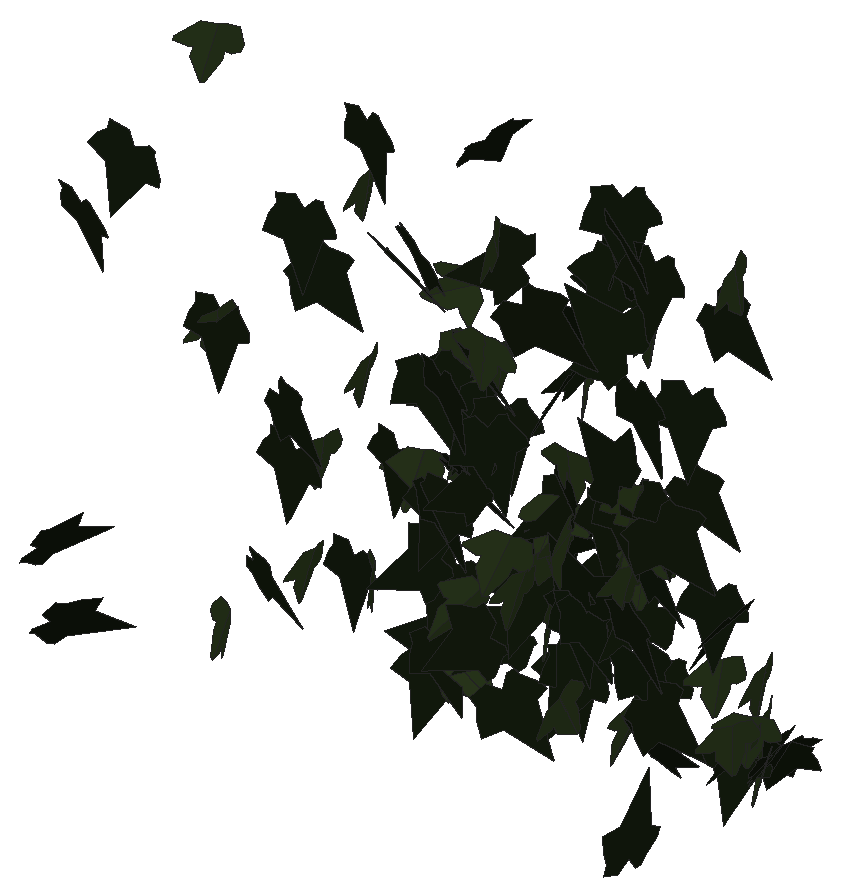
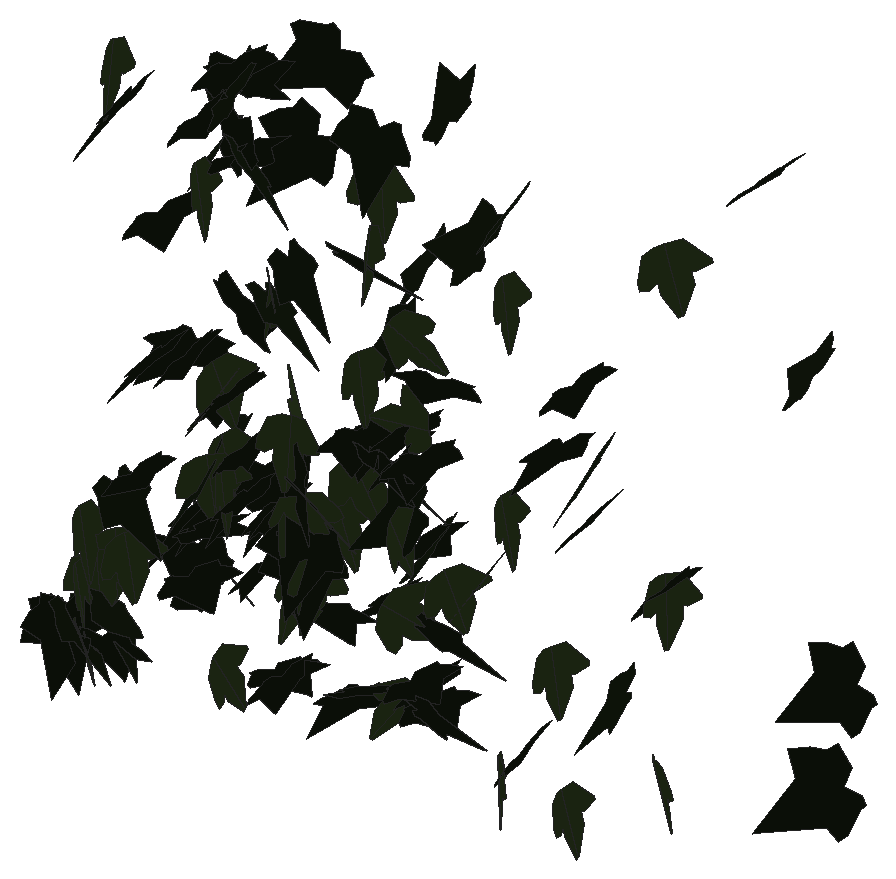
# SketchUp Ruby script. Lengths in inches.
U = 1.inch
M = Sketchup.active_model
def pt(a) = Geom::Point3d.new(a.map { |v| v * U })
def face(e, loops, mat)
  f = e.add_face(loops[0].map { |a| pt(a) })
  loops[1..].each { |l| e.add_face(l.map { |a| pt(a) }).erase! }
  f.material = f.back_material = mat if mat
  f
end
# faces: each face lists its corners as indices into pts; further lists are holes
def faces(e, pts, list, mat = nil) = list.each { |f| face(e, (f[0].is_a?(Array) ? f : [f]).map { |l| l.map { |i| pts[i] } }, mat) }
# xy, xz, yz: faces in a plane at the given z, y or x. An outline is a flat list of corners, or four numbers for a rectangle; further outlines are holes
def ring(l) = l.size == 4 ? [[l[0], l[1]], [l[2], l[1]], [l[2], l[3]], [l[0], l[3]]] : l.each_slice(2).to_a
def flat(e, list, mat, &to3) = list.each { |f| face(e, (f[0].is_a?(Array) ? f : [f]).map { |l| ring(l).map { |u, v| to3.(u, v) } }, mat) }
def xy(e, z, list, mat = nil) = flat(e, list, mat) { |x, y| [x, y, z] }
def xz(e, y, list, mat = nil) = flat(e, list, mat) { |x, z| [x, y, z] }
def yz(e, x, list, mat = nil) = flat(e, list, mat) { |y, z| [x, y, z] }
def lines(e, pts, list) = list.each { |a, b| e.add_line(pt(pts[a]), pt(pts[b])) }
# prism: a flat outline (further loops are holes) pulled along v
def prism(e, loops, v, mat = nil)
  f = face(e, loops, mat); d = Geom::Vector3d.new(v.map { |x| x * U })
  f.pushpull(f.normal.samedirection?(d) ? d.length : -d.length)
end
def box(e, o, s, mat = nil) = prism(e, [[o, [o[0] + s[0], o[1], o[2]], [o[0] + s[0], o[1] + s[1], o[2]], [o[0], o[1] + s[1], o[2]]]], [0, 0, s[2]], mat)
def at(x, y, z, deg = 0) = Geom::Transformation.translation(pt([x, y, z])) * Geom::Transformation.rotation(ORIGIN, Z_AXIS, deg.degrees)
def axes(o, x, y, z) = Geom::Transformation.new([*x, 0, *y, 0, *z, 0, *pt(o).to_a, 1])
def part(name) = M.definitions.add(name)
# library, detail: a bought-in or finely detailed component or shape, given as its bounding box
def library(name, o, s) = part(name).tap { |d| box(d.entities, o, s) }
def detail(e, o, s) = box(e.add_group.entities, o, s)
def put(e, d, t, mat = nil) = e.add_instance(d, t).tap { |i| i.material = mat if mat }
def group(e, t, mat = nil) = e.add_group.tap { |g| g.transformation = t; g.material = mat if mat }.entities
root = M.entities
M.materials.add("efeu1").color = [18, 25, 13]
M.materials.add("efeu2").color = [43, 57, 29]
c1 = part("ivyleaf_9")
p = [[1.54,2.16,1.25],[1.36,2.04,1.19],[-0.21,0.99,0.68],[-0.71,1.11,0.82],[-0.85,0.86,0.67],[-0.8,0.17,0.21],
  [-0.9,-0.01,0.1],[-0.67,-0.16,-0.02],[-0.08,-0.08,-0.05],[-0.03,-0.6,-0.4],[0.65,-0.88,-0.66],[0.83,-0.6,-0.49],
  [1.29,-0.42,-0.43],[1.8125,-0.07,-0.26],[1.21,0.44,0.15]]
faces(c1.entities,p,[[0,1,2,3,4,5,6,7,8,9,10,11,12,13,14]],"efeu1")
c2 = part("ivyleaf_10")
p = [[0,0.5,-0.03],[-0.0625,2.02,-0.43],[-0.19,2.01,-0.46],[-0.54,1.05,-0.29],[-0.52,0.625,-0.18],[-0.83,0.76,-0.28],
  [-1.16,0.64,-0.33],[-1.15,0.33,-0.24],[-0.77,-0.39,0.02],[-0.3,-0.51,0.16],[0.04,-0.48,0.23],[-0.02,2.01,-0.4375],
  [-0.06,2.01,-0.43],[0.04,-0.49,0.23],[0.67,-0.49,0.14],[1.38,0.36,-0.2],[1.375,0.51,-0.24],[0.81,0.65,-0.19],
  [0.62,0.59,-0.15],[0.6,1.09,-0.28],[0.5,1.23,-0.31]]
faces(c2.entities,p,[[0,1,2,3,4,5,6,7,8,9,10],[11,12,0,13,14,15,16,17,18,19,20]],"efeu2")
put(root,c1,axes([509.26,117.63,280.6],[0.7162,0.6229,0.94932],[0.53942,0.78067,-0.93141],[-1.06464,0.81457,0.1667]))
put(root,c1,axes([509.12,118.66,276.5],[0.94706,0.62855,0.77207],[0.59178,0.50664,-1.11926],[-0.868,1.03121,0.0793]))
put(root,c1,axes([509.17,120.39,295.65],[0.43222,-0.99904,0.53344],[0.29536,-0.45177,-1.08541],[1.09334,0.51698,0.08234]))
put(root,c2,axes([511.24,126.79,288.2],[-0.26325,-1.11937,-0.16844],[0.01435,0.16962,-1.14964],[1.13188,-0.26249,-0.0246]))
put(root,c1,axes([511.24,127.07,288.25],[0.01342,-1.16177,0.09011],[0.00969,-0.09,-1.16182],[1.16522,0.01413,0.00862]))
put(root,c2,axes([511.91,125.92,302.36],[-0.76297,-0.8833,0.30452],[-0.11819,-0.29874,-1.16269],[0.92681,-0.76525,0.10241]))
put(root,c1,axes([514.13,117.63,301.27],[-0.31009,-1.11283,0.47862],[0.13916,-0.5235,-1.12703],[1.20337,-0.22622,0.25366]))
put(root,c2,axes([514.92,122.69,276.87],[0.81565,-0.77415,-0.31621],[-0.18054,0.26829,-1.1225],[0.81652,0.83264,0.06768]))
put(root,c2,axes([515.36,127.93,277.68],[0.10975,-1.12799,0.06776],[0.00312,-0.06778,-1.13331],[1.13001,0.10974,-0.00345]))
put(root,c2,axes([516.27,127.56,283.53],[-0.20922,-1.13014,-0.01788],[-0.00453,0.01902,-1.14932],[1.13028,-0.20912,-0.00792]))
put(root,c1,axes([516.34,126.24,295.27],[-0.07104,-1.18727,-0.06644],[-0.00655,0.06695,-1.18934],[1.18911,-0.07057,-0.01052]))
put(root,c1,axes([516.54,122.875,279.96],[0.98177,-0.54869,-0.35898],[-0.27032,0.25016,-1.12167],[0.59737,1.01497,0.0824]))
put(root,c1,axes([516.66,126.62,292.67],[0.34915,-0.86934,-0.72445],[0.05079,0.76942,-0.89883],[1.13049,0.23392,0.26412]))
put(root,c1,axes([518.02,127.5,278.76],[0.17028,-1.0878,0.30446],[0.00985,-0.30645,-1.10045],[1.12956,0.16666,-0.0363]))
put(root,c2,axes([518.54,128.03,278.09],[0.66528,-0.87205,-0.28529],[0.0238,0.36868,-1.07143],[0.91722,0.62295,0.23473]))
put(root,c1,axes([518.7,121.82,289.12],[0.802,-0.75694,-0.50991],[-0.33518,0.3871,-1.10181],[0.84889,0.86797,0.04671]))
put(root,c2,axes([519.31,126.79,288.87],[0.23325,-1.14394,-0.09887],[-0.01611,0.09762,-1.16747],[1.14809,0.23378,0.0037]))
put(root,c1,axes([518.96,122.34,286.43],[-0.01682,-1.13373,0.40994],[0.11146,-0.40968,-1.12845],[1.2004,0.02215,0.11053]))
put(root,c2,axes([519.83,126.11,298.18],[0.19813,-1.16682,-0.20693],[-0.00093,0.20965,-1.18304],[1.18502,0.19525,0.03367]))
put(root,c1,axes([520.31,125.55,301.18],[0.43787,-1.1213,0.19248],[0.0419,-0.19021,-1.20339],[1.13693,0.43887,-0.02978]))
put(root,c1,axes([520.65,127.15,284.92],[0.11977,-1.02798,0.52313],[0.08685,-0.51641,-1.03466],[1.15016,0.14604,0.02366]))
put(root,c2,axes([521.81,127.17,284.89],[-0.57252,-0.9368,0.37642],[0.00691,-0.43636,-1.07545],[1.00957,-0.52826,0.22083]))
put(root,c1,axes([523.875,125.76,281.52],[-1.13577,0.158,0.39255],[-0.39229,0.02835,-1.14644],[-0.15863,-1.20136,0.02457]))
put(root,c1,axes([524.3,125.875,277.77],[-0.76854,0.43127,0.72687],[-0.6887,0.24993,-0.87647],[-0.48992,-1.02787,0.09185]))
put(root,c1,axes([523.35,127.53,280.19],[-0.45479,-1.05416,0.10034],[-0.0168,-0.102,-1.14781],[1.05879,-0.45442,0.02489]))
put(root,c1,axes([523.58,126.76,289.78],[-0.13333,-1.08675,-0.43796],[0.06968,0.43265,-1.09479],[1.1696,-0.14967,0.0153]))
put(root,c2,axes([524.9,126.27,294.68],[0.60536,0.03725,-1.03146],[-1.0202,0.2029,-0.59142],[0.15649,1.17864,0.13441]))
put(root,c1,axes([524.06,125.26,284.99],[0.67213,-1.01656,-0.05675],[-0.03339,0.04595,-1.21867],[1.0176,0.67296,-0.0025]))
put(root,c1,axes([523.74,122.79,297.39],[0.80288,-0.77938,0.55092],[0.51517,-0.25216,-1.10751],[0.80346,0.9405,0.1596]))
put(root,c2,axes([523.86,126.54,290.9375],[0.14036,0.03807,1.1742],[1.14694,0.25168,-0.14526],[-0.25444,1.15547,-0.00704]))
put(root,c2,axes([524.73,126.8,286.04],[0.2892,-1.04183,0.45253],[0.21949,-0.40691,-1.07707],[1.11446,0.3505,0.0947]))
put(root,c1,axes([524.32,126.5,290.7],[0.26155,-1.05452,-0.46703],[0.08644,0.49547,-1.07032],[1.15007,0.20258,0.18666]))
put(root,c1,axes([524.8,124.69,277.38],[-0.51302,-1.02415,0.01667],[-0.00704,-0.01512,-1.14546],[1.02427,-0.51307,0.00047]))
put(root,c1,axes([524.79,125.33,284.85],[-0.40551,-1.05086,0.29037],[-0.04899,-0.29193,-1.12492],[1.08914,-0.40439,0.05751]))
put(root,c1,axes([524.74,124.68,278.42],[0.24565,-1.06693,-0.34846],[-0.01246,0.35409,-1.09296],[1.12232,0.23746,0.06413]))
put(root,c1,axes([524.85,126.5,289.15],[0.12997,-1.16541,0.11002],[-0.01541,-0.11239,-1.17231],[1.17049,0.12793,-0.02765]))
put(root,c1,axes([524.79,124.22,291.67],[-0.36293,-0.93566,-0.71448],[0.73159,0.40652,-0.90398],[0.92234,-0.69061,0.43588]))
put(root,c1,axes([524.88,125.5,286.4],[1.16623,-0.32753,0.1954],[0.18385,-0.06798,-1.21125],[0.33415,1.18053,-0.01554]))
put(root,c1,axes([525.95,126.73,288.97],[-1.14286,-0.09267,-0.27996],[0.27902,0.02292,-1.14661],[0.09547,-1.17642,-0.00028]))
put(root,c2,axes([526.34,124.9,281.04],[-0.20033,-0.71324,0.96606],[-0.16303,-0.95419,-0.73828],[1.18971,-0.25086,0.0615]))
put(root,c2,axes([525.7,124.82,277.52],[0.4045,0.81164,0.72364],[0.33338,0.64234,-0.90681],[-1.03502,0.5241,-0.00927]))
put(root,c1,axes([526.79,127.25,278.38],[-0.94856,-0.49486,0.40687],[-0.13977,-0.54959,-0.99429],[0.62521,-0.87365,0.39501]))
put(root,c1,axes([526.74,125.47,302.7],[0.22673,1.19784,0.11087],[0.00467,0.11195,-1.219],[-1.20295,0.2262,0.01617]))
put(root,c1,axes([527.5,124.24,287.05],[-1.05091,0.44694,0.30048],[-0.28768,0.09112,-1.14167],[-0.45528,-1.08922,0.02779]))
put(root,c2,axes([526.95,126.25,292.39],[-0.09969,-1.18923,-0.09221],[0.01442,0.09133,-1.19339],[1.19272,-0.10051,0.00672]))
put(root,c2,axes([526.87,125.71,297.79],[0.39208,-1.0027,-0.54799],[0.03963,0.59093,-1.05292],[1.14198,0.32375,0.22468]))
put(root,c1,axes([526.34,124.44,293.24],[1.07571,-0.63641,-0.05333],[-0.04129,0.03493,-1.24984],[0.6373,1.07647,0.00903]))
put(root,c1,axes([527.97,126,296.88],[-1.01227,0.41714,0.51111],[-0.56307,-0.0585,-1.06745],[-0.34378,-1.13247,0.24341]))
put(root,c1,axes([527.1,126.27,289.44],[-0.26345,-1.07919,-0.40375],[0.10752,0.38934,-1.11082],[1.14722,-0.28432,0.01139]))
put(root,c1,axes([527.12,125.1,289.08],[-0.06933,-1.12895,-0.51525],[0.0311,0.51431,-1.13108],[1.24058,-0.07599,-0.00044]))
put(root,c1,axes([528.2,123.63,280.21],[-0.74453,-0.56698,0.78751],[-0.29754,-0.8114,-0.86549],[0.92364,-0.71842,0.35599]))
put(root,c1,axes([528.22,127,281.4375],[-0.86515,-0.74424,-0.24341],[0.27689,0.04853,-1.13253],[0.73245,-0.89743,0.14062]))
put(root,c1,axes([528.01,125.03,276.95],[0.2607,-0.89498,-0.76674],[0.20088,0.80754,-0.87429],[1.16126,0.06123,0.32337]))
put(root,c2,axes([528.68,126.96,282.85],[-0.33954,-1.03795,-0.42553],[0.12465,0.40694,-1.09205],[1.11485,-0.36162,-0.0075]))
put(root,c1,axes([527.97,119.51,300.22],[0.05578,-0.72625,1.04556],[0.47712,-0.95836,-0.69113],[1.18026,0.42174,0.22998]))
put(root,c1,axes([529.02,126.89,283.72],[0.49402,0.99682,-0.37978],[-0.13002,-0.35914,-1.11178],[-1.05876,0.50922,-0.04068]))
put(root,c1,axes([528.19,120.66,293.93],[0.55752,-1.04352,0.42032],[0.16487,-0.38825,-1.18259],[1.11285,0.58031,-0.03537]))
put(root,c1,axes([529.07,126.73,284.24],[0.68796,0.94268,-0.15589],[-0.11006,-0.11263,-1.16681],[-0.94913,0.69635,0.02231]))
put(root,c2,axes([529.47,126.7,285.44],[1.00994,0.49951,-0.35423],[-0.42659,0.08373,-1.09817],[-0.43933,1.06698,0.25201]))
put(root,c1,axes([530.01,126.53,286],[-1.11043,0.40907,0.08257],[-0.09083,-0.00782,-1.18275],[-0.40731,-1.11347,0.03864]))
put(root,c2,axes([529.69,123.08,285.35],[-0.81779,-0.78869,0.50414],[-0.22618,-0.48311,-1.12269],[0.90832,-0.83039,0.17434]))
put(root,c1,axes([530.1,126.55,287.15],[0.29638,0.01036,-1.15019],[-1.15016,0.01616,-0.29623],[0.01307,1.18766,0.01407]))
put(root,c2,axes([529.94,123.68,283.52],[0.00108,-1.16186,0.1635],[0.0034,-0.1635,-1.16186],[1.1733,0.00155,0.00322]))
put(root,c2,axes([529.97,126.73,284.53],[0.05845,-1.17459,0.00428],[-0.01828,-0.00519,-1.1759],[1.17445,0.05838,-0.01852]))
put(root,c1,axes([529.89,127.47,278.06],[0.00002,-1.13828,-0.18638],[-0.00846,0.18637,-1.13825],[1.15341,0.00139,-0.00835]))
put(root,c2,axes([530.51,126.37,288.34],[-1.17928,-0.06347,0.16864],[-0.16845,-0.00821,-1.18099],[0.06399,-1.19125,-0.00085]))
put(root,c1,axes([530.4,127.21,278.04],[-0.69121,-0.91987,0.0399],[0.04961,-0.08703,-1.14695],[0.9194,-0.68687,0.09189]))
put(root,c2,axes([530.92,120.2,296.68],[-1.17467,-0.14325,0.28175],[-0.27014,-0.10795,-1.18116],[0.1641,-1.20316,0.07243]))
put(root,c2,axes([530.68,124.92,282.23],[0.62617,-0.91261,0.47756],[0.35083,-0.3365,-1.10304],[0.96842,0.71199,0.09081]))
put(root,c1,axes([531.9375,125.8,293.63],[-0.81161,0.89778,0.03497],[-0.14537,-0.08472,-1.19902],[-0.88663,-0.80793,0.16458]))
put(root,c1,axes([531.16,127.02,282.49],[0.27296,-1.11304,-0.23533],[-0.00022,0.24196,-1.14464],[1.13765,0.26711,0.05624]))
put(root,c1,axes([532.49,123.75,294.1],[-0.6893,0.92152,-0.45373],[0.25844,-0.37326,-1.15069],[-0.99412,-0.73599,0.01546]))
put(root,c2,axes([531.98,125.73,293.66],[-0.59366,0.84866,-0.62841],[0.03235,-0.70595,-0.98394],[-1.0555,-0.49896,0.32329]))
put(root,c1,axes([533.125,124.15,283.2],[0.66071,0.00933,1.06659],[-1.00917,0.41171,0.62154],[-0.34537,-1.18518,0.22431]))
put(root,c1,axes([533.6,125.2,299.03],[-0.75465,0.87748,0.41902],[-0.29316,0.30042,-1.15709],[-0.92715,-0.80921,0.02481]))
put(root,c2,axes([532.96,122.67,279.1875],[-0.13058,-1.05676,-0.63879],[0.12852,0.62724,-1.06391],[1.22812,-0.178,0.04342]))
put(root,c1,axes([532.76,126.3125,286.76],[-0.03789,-1.17991,0.08695],[-0.0009,-0.08696,-1.18052],[1.18311,-0.03786,0.00189]))
put(root,c2,axes([532.63,122.88,286.19],[0.46324,-0.79609,-0.84419],[0.5024,-0.68176,0.91859],[-1.04595,-0.68004,0.06734]))
put(root,c1,axes([532.79,124.01,283.1],[0.22547,-1.15207,-0.01706],[-0.01626,0.0142,-1.17386],[1.15209,0.22567,-0.01323]))
put(root,c2,axes([533.375,126.92,276.95],[0.19764,-1.02003,0.48855],[0.06533,-0.48482,-1.03869],[1.1291,0.2066,-0.02541]))
put(root,c1,axes([532.97,124.06,283.18],[0.3968,-1.01679,-0.4335],[-0.13312,0.41328,-1.0912],[1.0973,0.41783,0.02438]))
put(root,c1,axes([532.97,125.86,284.45],[0.43745,-0.94854,-0.54517],[-0.10395,0.54844,-1.03764],[1.0891,0.43334,0.11993]))
put(root,c2,axes([533.59,126.54,285.19],[0.3257,-1.12558,-0.10672],[0.07669,0.1328,-1.16657],[1.12803,0.31596,0.11012]))
put(root,c1,axes([533.17,121.4375,298.4],[1.17151,0.49443,0.1404],[0.1358,0.03927,-1.27146],[-0.49572,1.17923,-0.01653]))
put(root,c1,axes([533.97,125.25,299.02],[-0.57954,-1.05101,0.26688],[0.01526,-0.31049,-1.18957],[1.08426,-0.55739,0.1594]))
put(root,c1,axes([533.71,125.3,299.05],[-0.19919,0.21932,1.19503],[0.61284,-1.02751,0.29073],[1.04911,0.64186,0.05706]))
put(root,c2,axes([534.61,126.26,285.1],[-0.84349,-0.7947,0.20262],[0.02056,-0.31106,-1.13442],[0.81987,-0.80979,0.23691]))
put(root,c1,axes([534.73,126.65,282.59],[-0.79584,-0.74014,0.43182],[-0.1423,-0.46699,-1.06269],[0.845,-0.77572,0.22773]))
put(root,c1,axes([535.53,123.17,290.45],[-0.14049,0.33413,1.23215],[-0.84015,0.90913,-0.34233],[-0.96123,-0.84345,0.11913]))
put(root,c1,axes([534.28,125.27,288.24],[0.15257,-1.17498,-0.12702],[0.00271,0.12842,-1.18469],[1.18183,0.15139,0.01912]))
put(root,c1,axes([534.45,124.91,302.68],[-0.14332,-1.18606,-0.3426],[0.04893,0.33917,-1.19466],[1.23358,-0.15126,0.00758]))
put(root,c2,axes([535,124.66,285.19],[-0.09662,-1.17079,0.08957],[-0.00954,-0.08909,-1.17477],[1.17417,-0.09706,-0.00218]))
put(root,c2,axes([535,125.13,288.68],[-0.29896,-1.08825,0.36496],[0.0334,-0.38523,-1.12132],[1.14733,-0.27235,0.12774]))
put(root,c1,axes([534.37,126.08,288.3],[0.52368,-1.06756,-0.00366],[0.00318,0.00564,-1.18908],[1.06756,0.52367,0.00534]))
put(root,c1,axes([534.27,125.02,301.49],[0.55156,-0.95488,0.56496],[0.28217,-0.48944,-1.10273],[1.07301,0.61954,-0.00041]))
put(root,c1,axes([534.67,125.99,285.23],[0.89539,-0.65015,-0.55073],[-0.42978,0.3452,-1.10627],[0.73571,0.99291,0.024]))
put(root,c1,axes([534.44,118.41,300.48],[-0.07794,-0.1337,-1.35641],[0.86357,1.04628,-0.15275],[1.0545,-0.86672,0.02484]))
put(root,c1,axes([535.33,126.41,280.12],[-0.54316,-1.01854,-0.09949],[0.01498,0.1047,-1.15376],[1.02328,-0.54218,-0.03591]))
put(root,c2,axes([535.83,125.24,297.27],[0.32748,-1.16403,-0.17268],[0.00525,0.18068,-1.20803],[1.17675,0.32313,0.05345]))
put(root,c1,axes([535.9,125.19,300.04],[-0.0501,-1.22395,0.12593],[-0.01957,-0.12522,-1.22489],[1.23025,-0.05183,-0.01436]))
put(root,c1,axes([535.96,123.16,284.26],[0.75817,-0.99098,0.08108],[0.04684,-0.06625,-1.24774],[0.99319,0.75961,-0.00305]))
put(root,c1,axes([536.21,123.6875,282.0625],[0.48598,-1.0285,-0.50939],[-0.11578,0.50642,-1.13297],[1.14188,0.48908,0.10192]))
put(root,c1,axes([536.61,125.15,289.03],[0.10647,-1.17955,0.09647],[-0.00118,-0.09697,-1.18431],[1.18349,0.10602,-0.00986]))
put(root,c1,axes([538.125,120.29,298.85],[-1.1158,-0.52246,-0.45001],[-0.4088,-0.18816,1.23206],[-0.5553,1.18833,-0.00277]))
put(root,c1,axes([537.08,126.15,289.56],[0.59935,-0.86466,-0.57736],[-0.08165,0.62522,-1.02109],[1.03649,0.54924,0.25342]))
put(root,c1,axes([536.77,123.67,278.18],[0.37109,-0.5199,1.09019],[0.89735,-0.6447,-0.6129],[0.80844,0.95425,0.17988]))
put(root,c2,axes([538.04,126.98,280.72],[-0.47803,-1.05017,0.1465],[0.05418,-0.18468,-1.14708],[1.05895,-0.46461,0.12482]))
put(root,c1,axes([537.73,127.04,284.16],[-0.12345,-1.16003,-0.05168],[0.00283,0.05167,-1.16658],[1.16118,-0.12345,-0.00265]))
put(root,c1,axes([537.375,123.66,288.81],[0.08245,-0.76755,-1.00995],[0.4399,0.96657,-0.69868],[1.1898,-0.30418,0.32831]))
put(root,c1,axes([538.55,126.87,283.25],[-0.52745,0.89287,-0.49278],[0.11625,-0.49852,-1.02772],[-1.01318,-0.52202,0.13861]))
put(root,c1,axes([537.7,122.66,280.87],[0.60019,-0.69605,-0.86478],[-0.25239,0.87177,-0.87685],[1.08103,0.58998,0.27541]))
put(root,c1,axes([538.24,124.71,294.66],[-0.22369,-1.18321,-0.17776],[0.01812,0.17747,-1.20407],[1.19635,-0.22392,-0.015]))
put(root,c1,axes([537.89,121.5,296.22],[0.57454,-1.15014,0.0967],[0.02675,-0.09472,-1.28553],[1.15389,0.57487,-0.01835]))
put(root,c1,axes([539.2,126.39,277.31],[-0.4076,1.02057,0.29385],[-0.21188,0.23028,-1.09368],[-1.04068,-0.44661,0.10758]))
put(root,c1,axes([538.59,127.76,276.83],[-0.86324,-0.58963,-0.44642],[0.43059,0.15716,-1.04021],[0.60129,-0.95905,0.104]))
put(root,c1,axes([539.39,119.14,275.78],[-1.11204,0.71545,-0.1428],[-0.11977,0.07776,1.32231],[0.71966,1.11847,-0.00059]))
put(root,c2,axes([539.73,127.78,276.71],[0.70891,-0.88264,0.03321],[0.01067,-0.03402,-1.13201],[0.8832,0.70887,-0.01298]))
put(root,c2,axes([540.04,126.43,279],[-0.93751,-0.63695,0.15688],[-0.12372,-0.09704,-1.13336],[0.64421,-0.94558,0.01063]))
put(root,c1,axes([540.45,127.49,277.37],[-0.677,0.90377,-0.17907],[0.04013,-0.19307,-1.12619],[-0.92046,-0.67314,0.0826]))
put(root,c2,axes([540,127.5,278.92],[0.43102,-1.05959,-0.14282],[0.01719,0.16084,-1.14137],[1.06903,0.42462,0.07594]))
put(root,c2,axes([540.15,127.0625,281.18],[0.2522,-1.20059,-0.14065],[0.00903,0.14554,-1.22619],[1.20877,0.24941,0.03851]))
put(root,c2,axes([540.23,124.97,279.28],[-0.55276,-1.0084,-0.08689],[0.04158,0.07629,-1.14996],[1.01128,-0.55432,-0.00021]))
put(root,c1,axes([540.5,127.86,277.46],[0.48334,0.75974,-0.69885],[-0.48016,-0.51763,-0.89483],[-0.91381,0.67385,0.10055]))
put(root,c1,axes([540.39,127.78,277.12],[0.29275,1.10256,0.05759],[-0.012,0.06275,-1.14043],[-1.104,0.29169,0.02766]))
put(root,c2,axes([540.23,125.08,301.16],[0.23749,-1.14417,-0.40361],[0.13553,0.43371,-1.14976],[1.20567,0.17662,0.20875]))
put(root,c1,axes([539.82,124.7,299.43],[0.72198,-0.80214,-0.70953],[-0.28057,0.68414,-1.05894],[1.03351,0.74608,0.20819]))
